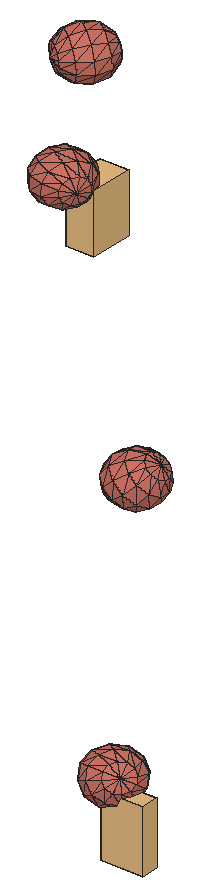
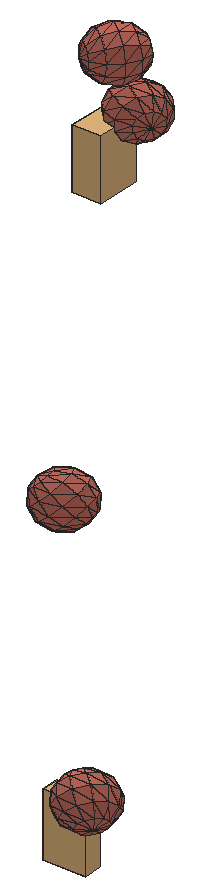
# SketchUp Ruby script. Lengths in inches.
U = 1.inch
M = Sketchup.active_model
def pt(a) = Geom::Point3d.new(a.map { |v| v * U })
def face(e, loops, mat)
  f = e.add_face(loops[0].map { |a| pt(a) })
  loops[1..].each { |l| e.add_face(l.map { |a| pt(a) }).erase! }
  f.material = f.back_material = mat if mat
  f
end
# faces: each face lists its corners as indices into pts; further lists are holes
def faces(e, pts, list, mat = nil) = list.each { |f| face(e, (f[0].is_a?(Array) ? f : [f]).map { |l| l.map { |i| pts[i] } }, mat) }
# xy, xz, yz: faces in a plane at the given z, y or x. An outline is a flat list of corners, or four numbers for a rectangle; further outlines are holes
def ring(l) = l.size == 4 ? [[l[0], l[1]], [l[2], l[1]], [l[2], l[3]], [l[0], l[3]]] : l.each_slice(2).to_a
def flat(e, list, mat, &to3) = list.each { |f| face(e, (f[0].is_a?(Array) ? f : [f]).map { |l| ring(l).map { |u, v| to3.(u, v) } }, mat) }
def xy(e, z, list, mat = nil) = flat(e, list, mat) { |x, y| [x, y, z] }
def xz(e, y, list, mat = nil) = flat(e, list, mat) { |x, z| [x, y, z] }
def yz(e, x, list, mat = nil) = flat(e, list, mat) { |y, z| [x, y, z] }
def lines(e, pts, list) = list.each { |a, b| e.add_line(pt(pts[a]), pt(pts[b])) }
# prism: a flat outline (further loops are holes) pulled along v
def prism(e, loops, v, mat = nil)
  f = face(e, loops, mat); d = Geom::Vector3d.new(v.map { |x| x * U })
  f.pushpull(f.normal.samedirection?(d) ? d.length : -d.length)
end
def box(e, o, s, mat = nil) = prism(e, [[o, [o[0] + s[0], o[1], o[2]], [o[0] + s[0], o[1] + s[1], o[2]], [o[0], o[1] + s[1], o[2]]]], [0, 0, s[2]], mat)
def at(x, y, z, deg = 0) = Geom::Transformation.translation(pt([x, y, z])) * Geom::Transformation.rotation(ORIGIN, Z_AXIS, deg.degrees)
def axes(o, x, y, z) = Geom::Transformation.new([*x, 0, *y, 0, *z, 0, *pt(o).to_a, 1])
def part(name) = M.definitions.add(name)
# library, detail: a bought-in or finely detailed component or shape, given as its bounding box
def library(name, o, s) = part(name).tap { |d| box(d.entities, o, s) }
def detail(e, o, s) = box(e.add_group.entities, o, s)
def put(e, d, t, mat = nil) = e.add_instance(d, t).tap { |i| i.material = mat if mat }
def group(e, t, mat = nil) = e.add_group.tap { |g| g.transformation = t; g.material = mat if mat }.entities
root = M.entities
M.materials.add("green").color = [174, 139, 102]
M.materials.add("vio").color = [206, 114, 100]
c1 = part("3DGeom~208_Defintion")
p = [[-278.9,104.85,-403.93],[-34.22,85.5625,-494.84],[-36.78,-106.97,-488.84],[218.15,-67.8125,-449.7],[219.62,43.35,-453.16],[33.05,253.77,-407.11],
  [-201.22,299.08,-302.625],[-278.9,104.85,-403.93],[-201.22,299.08,-302.625],[-281.85,-117.47,-397],[26.0625,-272.25,-390.72],[254.43,-163.24,-393.05],
  [-278.9,104.85,-403.93],[-281.85,-117.47,-397],[414.62,-10.48,-290.0625],[258.46,140.46,-402.51],[147.02,352.57,-249.16],[-69.62,413.17,-120.23],
  [33.05,253.77,-407.11],[-201.22,299.08,-302.625],[147.02,352.57,-249.16],[33.05,253.77,-407.11],[-448.85,96.04,-204.78],[-278.9,104.85,-403.93],
  [-281.85,-117.47,-397],[-381.57,264.25,-117.05],[-201.22,299.08,-302.625],[258.46,140.46,-402.51],[324.26,197.5,-311.32],[414.62,-10.48,-290.0625],
  [147.02,352.57,-249.16],[324.26,197.5,-311.32],[-451.4,-96.49,-198.78],[-209.29,-308.32,-283.69],[-281.85,-117.47,-397],[-209.29,-308.32,-283.69],
  [318.75,-217.36,-298.39],[318.75,-217.36,-298.39],[254.43,-163.24,-393.05],[414.62,-10.48,-290.0625],[-209.29,-308.32,-283.69],[26.0625,-272.25,-390.72],
  [137.48,-365.99,-226.76],[318.75,-217.36,-298.39],[137.48,-365.99,-226.76],[324.26,197.5,-311.32],[399.39,199.2,-204.01],[414.62,-10.48,-290.0625],
  [277.14,355.5,-63.3],[324.26,197.5,-311.32],[399.39,199.2,-204.01],[324.26,197.5,-311.32],[-267.6,363.06,40.9],[-201.22,299.08,-302.625],
  [-381.57,264.25,-117.05],[-267.6,363.06,40.9],[-201.22,299.08,-302.625],[318.75,-217.36,-298.39],[393.88,-215.66,-191.08],[393.88,-215.66,-191.08],
  [318.75,-217.36,-298.39],[414.62,-10.48,-290.0625],[459.68,-158.62,-99.89],[414.62,-10.48,-290.0625],[498.52,-61.5,-49.24],[414.62,-10.48,-290.0625],
  [500,49.66,-52.7],[414.62,-10.48,-290.0625],[399.39,199.2,-204.01],[463.72,145.08,-109.35],[414.62,-10.48,-290.0625],[414.62,-10.48,-290.0625],
  [-388.56,-261.77,-100.65],[-209.29,-308.32,-283.69],[-80.64,-416.55,-94.37],[-209.29,-308.32,-283.69],[-388.56,-261.77,-100.65],[80.64,416.55,94.37],
  [267.6,-363.06,-40.9],[393.88,-215.66,-191.08],[-498.52,61.5,49.24],[-459.68,158.62,99.89],[388.56,261.77,100.65],[399.39,199.2,-204.01],
  [388.56,261.77,100.65],[399.39,199.2,-204.01],[277.14,355.5,-63.3],[-500,-49.66,52.7],[267.6,-363.06,-40.9],[-137.48,365.99,226.76],
  [-267.6,363.06,40.9],[-393.88,215.66,191.08],[-267.6,363.06,40.9],[451.4,96.49,198.78],[388.56,261.77,100.65],[-388.56,-261.77,-100.65],
  [-277.14,-355.5,63.3],[-463.72,-145.08,109.35],[-277.14,-355.5,63.3],[267.6,-363.06,-40.9],[381.57,-264.25,117.05],[69.62,-413.17,120.23],
  [209.29,308.32,283.69],[388.56,261.77,100.65],[448.85,-96.04,204.78],[381.57,-264.25,117.05],[-318.75,217.36,298.39],[-267.6,363.06,40.9],
  [-393.88,215.66,191.08],[-318.75,217.36,298.39],[-267.6,363.06,40.9],[-414.62,10.48,290.0625],[-147.02,-352.57,249.16],[-277.14,-355.5,63.3],
  [-399.39,-199.2,204.01],[-399.39,-199.2,204.01],[-147.02,-352.57,249.16],[-26.0625,272.25,390.72],[-26.0625,272.25,390.72],[281.85,117.47,397],
  [388.56,261.77,100.65],[281.85,117.47,397],[388.56,261.77,100.65],[209.29,308.32,283.69],[381.57,-264.25,117.05],[201.22,-299.08,302.625],
  [201.22,-299.08,302.625],[-147.02,-352.57,249.16],[201.22,-299.08,302.625],[-318.75,217.36,298.39],[278.9,-104.85,403.93],[278.9,-104.85,403.93],
  [281.85,117.47,397],[-399.39,-199.2,204.01],[-147.02,-352.57,249.16],[-324.26,-197.5,311.32],[-324.26,-197.5,311.32],[201.22,-299.08,302.625],
  [278.9,-104.85,403.93],[-254.43,163.24,393.05],[-137.48,365.99,226.76],[-318.75,217.36,298.39],[-254.43,163.24,393.05],[-26.0625,272.25,390.72],
  [-137.48,365.99,226.76],[-324.26,-197.5,311.32],[-147.02,-352.57,249.16],[-33.05,-253.77,407.11],[-147.02,-352.57,249.16],[201.22,-299.08,302.625],
  [-33.05,-253.77,407.11],[36.78,106.98,488.84],[209.29,308.32,283.69],[281.85,117.47,397],[209.29,308.32,283.69],[-258.46,-140.46,402.51],
  [-258.46,-140.46,402.51],[-219.62,-43.35,453.16],[-414.62,10.48,290.0625],[-218.15,67.8125,449.7],[-414.62,10.48,290.0625],[-254.43,163.24,393.05],
  [-254.43,163.24,393.05],[-414.62,10.48,290.0625],[201.22,-299.08,302.625],[278.9,-104.85,403.93],[-324.26,-197.5,311.32],[-254.43,163.24,393.05],
  [34.22,-85.5625,494.84]]
faces(c1.entities,p,[[0,1,2],[1,3,2],[1,4,3],[5,4,1],[6,1,7],[8,5,1],[9,2,10],[2,11,10],
  [2,3,11],[12,2,13],[3,4,14],[4,15,14],[5,15,4],[11,3,14],[16,15,5],[17,18,19],
  [17,20,21],[22,23,24],[25,23,22],[25,26,23],[27,28,29],[30,31,15],[32,24,33],[34,10,35],
  [22,24,32],[10,11,36],[37,38,39],[40,41,42],[10,43,44],[45,46,47],[48,49,20],[48,50,51],
  [52,53,54],[55,17,56],[42,57,58],[59,60,61],[62,59,63],[64,62,65],[66,64,67],[68,69,70],
  [69,66,71],[72,73,74],[75,42,74],[32,33,76],[77,20,17],[77,48,20],[74,42,78],[42,79,78],
  [80,22,32],[81,22,80],[81,25,22],[82,69,83],[84,85,86],[87,32,76],[80,32,87],[88,59,62],
  [89,17,90],[89,77,17],[91,25,81],[91,92,25],[93,66,69],[93,69,94],[95,74,96],[97,76,98],
  [87,76,97],[99,62,100],[100,62,64],[96,74,101],[74,78,101],[102,103,48],[102,48,77],[104,64,66],
  [104,66,93],[100,64,104],[101,78,105],[106,107,108],[109,89,110],[80,87,111],[81,80,111],[87,97,111],
  [96,101,112],[97,113,114],[115,96,116],[117,77,89],[118,102,77],[91,81,111],[119,93,120],[121,122,123],
  [97,114,111],[101,124,125],[126,100,104],[127,101,128],[129,91,111],[130,104,93],[131,93,132],[133,134,135],
  [114,136,111],[137,104,138],[139,140,141],[142,143,144],[145,146,147],[148,149,150],[151,152,143],[151,153,154],
  [136,155,111],[156,157,158],[157,159,160],[161,129,111],[159,162,163],[147,164,165],[166,147,156],[159,143,167],
  [159,151,143],[168,165,153],[168,153,151],[156,147,168],[156,168,157],[147,165,168],[157,151,159],[157,168,151]],"vio")
c2 = part("3DGeom~244_Defintion")
p = [[-108.99,-83.02,-483.7],[90.05,60.9,-492.09],[201.25,-102.35,-447.625],[393.37,0,-317.28],[-208.69,-14.03,-459.98],[-82.63,180.41,-451.01],
  [264.97,188.51,-368.625],[-44.79,-177.28,-458.03],[-278.83,-204.71,-345.7],[-317.18,11.23,-393.23],[-33.3,-271.53,-389.85],[221.17,-265.61,-329.54],
  [221.17,-265.61,-329.54],[-270.53,224.16,-335.4],[65.57,326.51,-321.2],[416.36,-188.51,-180.93],[221.17,-265.61,-329.54],[416.36,-188.51,-180.93],
  [-405.375,-14.03,-301.34],[-405.375,-14.03,-301.34],[-270.53,224.16,-335.4],[-317.18,11.23,-393.23],[-33.3,-271.53,-389.85],[144.46,-385.12,-169.46],
  [-77.58,-340.53,-297.43],[-33.3,-271.53,-389.85],[221.17,-265.61,-329.54],[-77.58,-340.53,-297.43],[264.97,188.51,-368.625],[480.09,102.35,-101.93],
  [393.37,0,-317.28],[264.97,188.51,-368.625],[368.89,265.61,-146.39],[65.57,326.51,-321.2],[368.89,265.61,-146.39],[264.97,188.51,-368.625],
  [-165.78,-365.79,-205.53],[-165.78,-365.79,-205.53],[-274.26,-340.53,-138.79],[-278.83,-204.71,-345.7],[-274.26,-340.53,-138.79],[-373.96,-271.53,-115.07],
  [-278.83,-204.71,-345.7],[-438.16,-177.28,-140.74],[-278.83,-204.71,-345.7],[-449.66,-83.02,-208.92],[-405.375,-14.03,-301.34],[-278.83,-204.71,-345.7],
  [-278.83,-204.71,-345.7],[-405.375,-14.03,-301.34],[-423.3,180.41,-176.24],[-270.53,224.16,-335.4],[-151.39,377.02,-187.7],[-270.53,224.16,-335.4],
  [-151.39,377.02,-187.7],[327.8,-326.51,3.91],[416.36,-188.51,-180.93],[65.57,326.51,-321.2],[196.2,385.12,-105.3125],[368.89,265.61,-146.39],
  [-151.39,377.02,-187.7],[65.57,326.51,-321.2],[393.37,0,-317.28],[500,-60.9,16.16],[416.36,-188.51,-180.93],[393.37,0,-317.28],
  [-405.375,-14.03,-301.34],[-77.58,-340.53,-297.43],[-8.31,-428.86,-10.3],[-165.78,-365.79,-205.53],[-77.58,-340.53,-297.43],[-500,60.9,-16.16],
  [-165.78,-365.79,-205.53],[-196.2,-385.12,105.3125],[-165.78,-365.79,-205.53],[-274.26,-340.53,-138.79],[-327.8,326.51,-3.91],[-151.39,377.02,-187.7],
  [-327.8,326.51,-3.91],[8.31,428.86,10.3],[-151.39,377.02,-187.7],[-151.39,377.02,-187.7],[416.36,-188.51,-180.93],[423.3,-180.41,176.24],
  [327.8,-326.51,3.91],[416.36,-188.51,-180.93],[151.39,-377.02,187.7],[438.16,177.28,140.74],[373.96,271.53,115.07],[373.96,271.53,115.07],
  [368.89,265.61,-146.39],[-480.09,-102.35,101.93],[-274.26,-340.53,-138.79],[-368.89,-265.61,146.39],[-274.26,-340.53,-138.79],[-368.89,-265.61,146.39],
  [-373.96,-271.53,-115.07],[-368.89,-265.61,146.39],[274.26,340.53,138.79],[373.96,271.53,115.07],[449.66,83.02,208.92],[-416.36,188.51,180.93],
  [-65.57,-326.51,321.2],[-416.36,188.51,180.93],[-144.46,385.12,169.46],[-327.8,326.51,-3.91],[-327.8,326.51,-3.91],[327.8,-326.51,3.91],
  [270.53,-224.16,335.4],[151.39,-377.02,187.7],[327.8,-326.51,3.91],[165.78,365.79,205.53],[405.375,14.03,301.34],[-393.37,0,317.28],
  [-264.97,-188.51,368.625],[-368.89,-265.61,146.39],[-264.97,-188.51,368.625],[278.83,204.71,345.7],[274.26,340.53,138.79],[278.83,204.71,345.7],
  [278.83,204.71,345.7],[278.83,204.71,345.7],[-264.97,-188.51,368.625],[-416.36,188.51,180.93],[-221.17,265.61,329.54],[77.58,340.54,297.43],
  [317.18,-11.23,393.23],[-393.37,0,317.28],[-221.17,265.61,329.54],[-416.36,188.51,180.93],[151.39,-377.02,187.7],[82.63,-180.41,451.01],
  [-65.57,-326.51,321.2],[151.39,-377.02,187.7],[270.53,-224.16,335.4],[165.78,365.79,205.53],[77.58,340.54,297.43],[278.83,204.71,345.7],
  [278.83,204.71,345.7],[77.58,340.54,297.43],[33.3,271.53,389.85],[33.3,271.53,389.85],[317.18,-11.23,393.23],[405.375,14.03,301.34],
  [-264.97,-188.51,368.625],[-201.25,102.35,447.625],[-393.37,0,317.28],[-393.37,0,317.28],[-221.17,265.61,329.54],[-65.57,-326.51,321.2],
  [-90.05,-60.9,492.09],[-264.97,-188.51,368.625],[-65.57,-326.51,321.2],[33.3,271.53,389.85],[-221.17,265.61,329.54],[270.53,-224.16,335.4],
  [208.69,14.03,459.98],[270.53,-224.16,335.4],[317.18,-11.23,393.23],[317.18,-11.23,393.23],[108.99,83.02,483.7],[44.79,177.28,458.03],
  [33.3,271.53,389.85],[-264.97,-188.51,368.625],[33.3,271.53,389.85]]
faces(c2.entities,p,[[0,1,2],[1,3,2],[4,1,0],[4,5,1],[1,6,3],[5,6,1],[0,7,8],[4,0,8],
  [0,2,7],[9,4,8],[9,5,4],[7,10,8],[7,11,10],[7,2,12],[9,13,5],[13,14,5],
  [5,14,6],[2,15,16],[2,3,17],[18,9,8],[19,20,21],[22,23,24],[25,26,23],[10,27,8],
  [28,29,30],[31,32,29],[33,34,35],[27,36,8],[37,38,39],[40,41,42],[41,43,44],[45,46,47],
  [43,45,48],[49,50,51],[50,52,53],[13,54,14],[26,55,23],[26,56,55],[57,58,59],[60,58,61],
  [62,63,64],[65,29,63],[45,50,66],[67,68,69],[70,23,68],[43,71,45],[45,71,50],[72,68,73],
  [74,73,75],[50,76,77],[78,79,80],[81,79,58],[82,83,84],[85,63,83],[71,76,50],[23,86,68],
  [23,55,86],[32,87,29],[32,88,87],[58,89,90],[41,91,43],[43,91,71],[92,73,93],[94,95,96],
  [41,97,91],[58,98,99],[79,98,58],[29,100,63],[29,87,100],[91,101,71],[71,101,76],[68,102,73],
  [68,86,102],[103,104,105],[106,104,79],[107,108,109],[110,83,108],[79,111,98],[104,111,79],[63,112,83],
  [63,100,112],[97,113,91],[91,113,101],[73,114,115],[73,102,116],[87,88,117],[88,118,119],[98,111,120],
  [100,87,121],[97,122,113],[123,124,104],[124,125,104],[104,125,111],[83,126,108],[83,112,126],[127,128,129],
  [130,131,132],[133,134,131],[135,136,137],[112,100,138],[139,140,137],[124,141,125],[142,143,137],[144,145,146],
  [147,145,148],[149,150,151],[152,131,150],[145,153,154],[155,156,131],[157,158,156],[156,159,137],[160,156,137],
  [161,160,137],[162,161,137],[163,150,145],[145,161,164],[150,161,145],[131,160,150],[131,156,160],[150,160,161]],"vio")
c3 = part("3DGeom~248_Defintion")
p = [[242.2,-95.53,-426.77],[-5.12,-61.18,-498.23],[-8.42,49.39,-500],[242.2,-95.53,-426.77],[236.48,95.97,-429.83],[-251.07,-10.43,-436.2],
  [-67.73,144.3,-469.01],[149.39,-262.83,-367.79],[-58.71,-157.77,-464.19],[242.2,-95.53,-426.77],[-167.15,198.125,-413.57],[133.76,260.36,-376.15],
  [133.76,260.36,-376.15],[-17.09,-361.11,-268.71],[-154.82,-214.51,-406.98],[-17.09,-361.11,-268.71],[-267.71,-216.1875,-341.94],[-367.14,-162.36,-286.51],
  [-267.71,-216.1875,-341.94],[-367.14,-162.36,-286.51],[-426.44,-67.45,-255.52],[-426.44,-67.45,-255.52],[-429.75,43.11,-257.28],[-251.07,-10.43,-436.2],
  [-429.75,43.11,-257.28],[-376.16,139.71,-291.33],[-376.16,139.71,-291.33],[-280.04,196.44,-348.54],[-280.04,196.44,-348.54],[424.625,-104.29,-240.95],
  [242.2,-95.53,-426.77],[236.48,95.97,-429.83],[236.48,95.97,-429.83],[418.02,116.84,-244.48],[418.02,116.84,-244.48],[133.76,260.36,-376.15],
  [317.45,-297.47,-172.85],[242.2,-95.53,-426.77],[317.45,-297.47,-172.85],[242.2,-95.53,-426.77],[424.625,-104.29,-240.95],[-38.44,353.59,-280.13],
  [-280.04,196.44,-348.54],[133.76,260.36,-376.15],[-38.44,353.59,-280.13],[-212.625,-364.02,-156.07],[-267.71,-216.1875,-341.94],[-154.82,-214.51,-406.98],
  [-154.82,-214.51,-406.98],[-17.09,-361.11,-268.71],[418.02,116.84,-244.48],[133.76,260.36,-376.15],[299.4,306.66,-182.51],[299.4,306.66,-182.51],
  [133.76,260.36,-376.15],[-38.44,353.59,-280.13],[125.22,-410.95,-58.44],[149.39,-262.83,-367.79],[149.39,-262.83,-367.79],[317.45,-297.47,-172.85],
  [-233.98,350.68,-167.49],[-280.04,196.44,-348.54],[-376.16,139.71,-291.33],[-38.44,353.59,-280.13],[-280.04,196.44,-348.54],[-233.98,350.68,-167.49],
  [-384.83,-270.79,-60.04],[-267.71,-216.1875,-341.94],[-212.625,-364.02,-156.07],[-367.14,-162.36,-286.51],[-267.71,-216.1875,-341.94],[-400.46,252.4,-68.4],
  [-233.98,350.68,-167.49],[-487.55,-106.4,-6.37],[100.5625,414.3125,-71.63],[-233.98,350.68,-167.49],[-100.5625,-414.3125,71.63],[-493.27,85.1,-9.43],
  [493.27,-85.1,9.43],[487.55,106.4,6.37],[299.4,306.66,-182.51],[400.46,-252.4,68.4],[317.45,-297.47,-172.85],[299.4,306.66,-182.51],
  [384.83,270.79,60.04],[384.83,270.79,60.04],[233.98,-350.68,167.49],[317.45,-297.47,-172.85],[233.98,-350.68,167.49],[317.45,-297.47,-172.85],
  [400.46,-252.4,68.4],[-125.22,410.95,58.44],[-400.46,252.4,-68.4],[-299.4,-306.66,182.51],[-299.4,-306.66,182.51],[-384.83,-270.79,-60.04],
  [384.83,270.79,60.04],[212.625,364.02,156.07],[-317.45,297.47,172.85],[-400.46,252.4,-68.4],[-317.45,297.47,172.85],[-418.02,-116.84,244.48],
  [-299.4,-306.66,182.51],[-418.02,-116.84,244.48],[38.44,-353.59,280.13],[38.44,-353.59,280.13],[233.98,-350.68,167.49],[-424.625,104.29,240.95],
  [-317.45,297.47,172.85],[-418.02,-116.84,244.48],[429.75,-43.11,257.28],[426.44,67.45,255.52],[426.44,67.45,255.52],[376.16,-139.71,291.33],
  [376.16,-139.71,291.33],[17.09,361.11,268.71],[-317.45,297.47,172.85],[17.09,361.11,268.71],[426.44,67.45,255.52],[367.14,162.36,286.51],
  [367.14,162.36,286.51],[212.625,364.02,156.07],[280.04,-196.44,348.54],[233.98,-350.68,167.49],[280.04,-196.44,348.54],[376.16,-139.71,291.33],
  [-133.76,-260.36,376.15],[-299.4,-306.66,182.51],[-133.76,-260.36,376.15],[38.44,-353.59,280.13],[367.14,162.36,286.51],[212.625,364.02,156.07],
  [267.71,216.1875,341.94],[267.71,216.1875,341.94],[17.09,361.11,268.71],[167.15,-198.125,413.57],[38.44,-353.59,280.13],[233.98,-350.68,167.49],
  [233.98,-350.68,167.49],[280.04,-196.44,348.54],[-149.39,262.83,367.79],[-317.45,297.47,172.85],[-424.625,104.29,240.95],[17.09,361.11,268.71],
  [-317.45,297.47,172.85],[-149.39,262.83,367.79],[-236.48,-95.97,429.83],[-418.02,-116.84,244.48],[-299.4,-306.66,182.51],[-133.76,-260.36,376.15],
  [-242.2,95.53,426.77],[-418.02,-116.84,244.48],[-424.625,104.29,240.95],[-242.2,95.53,426.77],[-242.2,95.53,426.77],[-418.02,-116.84,244.48],
  [-236.48,-95.97,429.83],[426.44,67.45,255.52],[251.07,10.43,436.2],[426.44,67.45,255.52],[367.14,162.36,286.51],[251.07,10.43,436.2],
  [376.16,-139.71,291.33],[429.75,-43.11,257.28],[154.82,214.51,406.98],[17.09,361.11,268.71],[267.71,216.1875,341.94],[17.09,361.11,268.71],
  [154.82,214.51,406.98],[67.73,-144.3,469.01],[267.71,216.1875,341.94],[58.71,157.77,464.19],[8.42,-49.39,500],[5.12,61.18,498.23]]
faces(c3.entities,p,[[0,1,2],[3,2,4],[2,1,5],[6,2,5],[4,2,6],[7,8,1],[7,1,9],[1,8,5],
  [10,6,5],[4,6,11],[12,6,10],[13,14,8],[15,8,7],[8,14,5],[16,17,5],[14,18,5],
  [19,20,5],[21,22,23],[24,25,5],[26,27,5],[28,10,5],[29,30,31],[29,32,33],[34,4,35],
  [36,7,37],[38,39,40],[41,10,42],[43,10,44],[45,46,47],[45,48,49],[50,51,52],[53,54,55],
  [56,49,57],[56,58,59],[60,61,62],[63,64,65],[66,67,68],[66,69,70],[71,62,22],[72,62,71],
  [73,69,66],[73,21,69],[53,55,74],[74,55,75],[76,45,49],[76,49,56],[77,22,21],[71,22,77],
  [77,21,73],[78,29,33],[78,33,79],[79,33,80],[81,82,29],[81,29,78],[79,83,84],[85,53,74],
  [86,56,87],[88,89,90],[91,75,92],[74,75,91],[93,45,76],[94,95,45],[96,74,97],[97,74,91],
  [98,71,77],[91,99,100],[101,66,102],[103,73,66],[104,76,56],[105,56,106],[107,77,73],[108,77,107],
  [107,73,109],[110,78,79],[110,79,111],[112,79,84],[113,81,78],[114,78,110],[115,91,116],[97,91,117],
  [118,84,119],[120,84,121],[122,123,81],[124,81,125],[126,127,76],[128,76,129],[130,131,132],[133,97,134],
  [135,136,137],[135,138,139],[140,141,142],[143,144,145],[146,147,148],[146,148,149],[150,107,151],[140,152,153],
  [154,155,156],[110,157,158],[159,160,161],[162,163,161],[164,165,140],[166,167,168],[169,149,136],[169,136,135],
  [160,170,161],[139,162,161],[170,164,161],[135,139,161],[171,140,153],[164,140,171],[172,146,149],[172,149,169],
  [164,171,161],[169,135,161],[173,153,146],[171,153,173],[173,146,172],[172,169,161],[173,172,161],[171,173,161]],"vio")
c4 = part("3DGeom~241_Defintion")
p = [[-83.63,87.77,-500],[-95.35,-182.17,-461.02],[-273.19,-13.21,-439.1],[14.09,-123.87,-496.18],[142.8125,124.74,-475.08],[-158.95,275.9,-369.85],
  [-273.19,-13.21,-439.1],[102.53,318.58,-341.07],[-158.95,275.9,-369.85],[102.53,318.58,-341.07],[108.04,-302.32,-359.41],[144.83,-102.53,-481.79],
  [108.04,-302.32,-359.41],[261.83,-123.87,-421.71],[108.04,-302.32,-359.41],[345.47,87.77,-371.01],[336.53,275.9,-220.9],[336.53,275.9,-220.9],
  [102.53,318.58,-341.07],[-154.17,-261.82,-385.73],[108.04,-302.32,-359.41],[-273.19,-13.21,-439.1],[-273.19,-13.21,-439.1],[-375.08,-151.16,-308.7],
  [-377.83,159.29,-299.52],[-273.19,-13.21,-439.1],[-375.08,-151.16,-308.7],[-158.95,275.9,-369.85],[-273.19,-13.21,-439.1],[-377.83,159.29,-299.52],
  [333.75,-182.17,-332.03],[108.04,-302.32,-359.41],[470.03,-13.21,-215.68],[333.75,-182.17,-332.03],[261.83,-123.87,-421.71],[261.83,-123.87,-421.71],
  [345.47,87.77,-371.01],[-375.08,-151.16,-308.7],[-146.61,-341.47,-290.49],[-146.61,-341.47,-290.49],[108.04,-302.32,-359.41],[480.36,159.29,-41.54],
  [345.47,87.77,-371.01],[345.47,87.77,-371.01],[336.53,275.9,-220.9],[-191.67,390.1,-140.59],[-158.95,275.9,-369.85],[34.77,427.0625,-115.67],
  [-158.95,275.9,-369.85],[-191.67,390.1,-140.59],[102.53,318.58,-341.07],[-158.95,275.9,-369.85],[42.3,-421.11,-140.72],[-74.7,-399.77,-200.81],
  [108.04,-302.32,-359.41],[173.04,-399.77,-126.33],[-146.61,-341.47,-290.49],[282.49,-341.47,-161.49],[341.31,-261.82,-236.78],[282.49,-341.47,-161.49],
  [333.75,-182.17,-332.03],[341.31,-261.82,-236.78],[108.04,-302.32,-359.41],[237.42,390.1,-11.6],[336.53,275.9,-220.9],[483.12,-151.16,-50.71],
  [341.31,-261.82,-236.78],[-375.08,-151.16,-308.7],[-146.61,-341.47,-290.49],[-361.98,-289.11,-143.73],[-495.48,0,-148.95],[-361.98,-289.11,-143.73],
  [-381.24,289.11,-79.69],[-191.67,390.1,-140.59],[-361.98,-289.11,-143.73],[381.24,-289.11,79.69],[282.49,-341.47,-161.49],[361.98,289.11,143.73],
  [336.53,275.9,-220.9],[361.98,289.11,143.73],[336.53,275.9,-220.9],[237.42,390.1,-11.6],[495.48,0,148.95],[-237.42,-390.1,11.6],
  [-361.98,-289.11,-143.73],[191.67,-390.1,140.59],[282.49,-341.47,-161.49],[191.67,-390.1,140.59],[282.49,-341.47,-161.49],[381.24,-289.11,79.69],
  [-480.36,-159.29,41.54],[-483.12,151.16,50.71],[-237.42,-390.1,11.6],[-34.77,-427.0625,115.67],[-173.04,399.77,126.33],[-381.24,289.11,-79.69],
  [-42.3,421.11,140.72],[191.67,-390.1,140.59],[74.7,399.77,200.81],[-282.49,341.47,161.5],[-381.24,289.11,-79.69],[-282.49,341.47,161.5],
  [377.83,-159.29,299.53],[375.08,151.16,308.7],[375.08,151.16,308.7],[361.98,289.11,143.73],[146.61,341.47,290.49],[361.98,289.11,143.73],
  [-336.53,-275.9,220.9],[-237.42,-390.1,11.6],[-336.53,-275.9,220.9],[-470.03,13.21,215.68],[-336.53,-275.9,220.9],[-341.31,261.82,236.78],
  [-282.49,341.47,161.5],[-341.31,261.82,236.78],[158.95,-275.9,369.85],[191.67,-390.1,140.59],[158.95,-275.9,369.85],[-336.53,-275.9,220.9],
  [-102.53,-318.58,341.07],[-102.53,-318.58,341.07],[191.67,-390.1,140.59],[-108.04,302.32,359.41],[-108.04,302.32,359.41],[-102.53,-318.58,341.07],
  [191.67,-390.1,140.59],[158.95,-275.9,369.85],[-108.04,302.32,359.41],[154.17,261.82,385.73],[375.08,151.16,308.7],[361.98,289.11,143.73],
  [361.98,289.11,143.73],[146.61,341.47,290.49],[273.19,13.21,439.1],[273.19,13.21,439.1],[375.08,151.16,308.7],[-341.31,261.82,236.78],
  [-108.04,302.32,359.41],[-108.04,302.32,359.41],[-336.53,-275.9,220.9],[-345.47,-87.77,371.01],[-333.75,182.17,332.03],[-345.47,-87.77,371.01],
  [-341.31,261.82,236.78],[-333.75,182.17,332.03],[-345.47,-87.77,371.01],[-336.53,-275.9,220.9],[-102.53,-318.58,341.07],[-341.31,261.82,236.78],
  [-333.75,182.17,332.03],[-108.04,302.32,359.41],[146.61,341.47,290.49],[83.63,-87.77,500],[158.95,-275.9,369.85],[377.83,-159.29,299.53],
  [377.83,-159.29,299.53],[273.19,13.21,439.1],[95.35,182.17,461.02],[-333.75,182.17,332.03],[-345.47,-87.77,371.01],[-261.83,123.87,421.71],
  [-261.83,123.87,421.71],[-142.8125,-124.74,475.08],[-144.83,102.53,481.79],[-14.09,123.87,496.18]]
faces(c4.entities,p,[[0,1,2],[0,3,1],[4,3,0],[5,0,6],[7,0,8],[9,4,0],[1,3,10],[3,11,12],
  [4,11,3],[11,13,14],[15,13,11],[15,11,4],[16,15,4],[17,4,18],[19,1,20],[21,1,19],
  [22,19,23],[24,25,26],[27,28,29],[13,30,31],[32,33,34],[32,35,36],[37,19,38],[39,19,40],
  [41,32,42],[41,43,44],[45,46,24],[47,48,49],[47,50,51],[52,53,54],[55,52,54],[53,56,54],
  [57,55,54],[58,59,54],[60,61,62],[63,64,50],[63,50,47],[65,66,33],[65,33,32],[67,68,69],
  [70,26,71],[24,26,70],[72,24,70],[73,24,72],[74,56,53],[75,76,66],[75,66,65],[77,41,78],
  [79,80,81],[82,65,32],[82,32,41],[83,53,52],[84,53,83],[85,55,86],[87,88,89],[70,71,90],
  [91,70,90],[72,70,91],[90,71,92],[83,52,93],[93,52,55],[94,49,95],[96,47,49],[96,49,94],
  [93,55,97],[98,63,47],[98,47,96],[99,72,91],[94,100,101],[102,75,65],[102,65,82],[103,82,41],
  [104,41,105],[106,107,63],[106,63,98],[108,83,93],[90,109,110],[111,90,112],[91,90,111],[113,91,111],
  [114,91,115],[116,117,75],[118,75,102],[119,93,120],[121,93,122],[94,101,123],[96,94,124],[125,126,127],
  [98,96,128],[129,130,131],[129,132,133],[134,102,82],[135,82,136],[101,137,138],[106,98,139],[111,140,141],
  [142,111,143],[144,111,145],[146,147,148],[149,150,151],[129,152,151],[153,154,155],[153,156,157],[158,157,130],
  [158,130,129],[159,160,161],[150,162,151],[146,148,163],[163,148,154],[162,164,151],[164,165,151],[165,158,151],
  [158,129,151],[163,154,153],[162,146,163],[162,163,164],[165,153,157],[165,157,158],[164,163,153],[164,153,165]],"vio")
c5 = library("3DGeom~173_Defintion",[-146.02,-500,-341.01],[292.04,1000,682.02])
c6 = part("3DGeom~174_Defintion")
p = [[-127.07,494.74,-302.98],[-83.38,461.51,-336.48],[-100.9,461.46,-341.01],[-127.07,494.74,-302.98],[-117.78,466.57,-338.44],[-127.07,494.74,-302.98],
  [-117.78,466.57,-338.44],[-129.48,475.47,-329.47],[-127.07,494.74,-302.98],[-69.91,466.72,-326.0625],[-127.07,494.74,-302.98],[-129.48,475.47,-329.47],
  [-132.89,485.78,-316.49],[-127.07,494.74,-302.98],[-64.09,475.68,-312.56],[-69.91,466.72,-326.0625],[-127.07,494.74,-302.98],[-67.49,485.99,-299.58],
  [-64.09,475.68,-312.56],[-127.07,494.74,-302.98],[-79.2,494.89,-290.61],[-67.49,485.99,-299.58],[-127.07,494.74,-302.98],[-113.59,499.94,-292.57],
  [-96.07,500,-288.04],[-127.07,494.74,-302.98],[-96.07,500,-288.04],[-79.2,494.89,-290.61],[109.52,-498.77,278.33],[81.81,-497.43,299.58],
  [93.08,-500,285.75],[109.52,-498.77,278.33],[84.66,-484.5,330.92],[81.81,-497.43,299.58],[140.09,-487.18,288.41],[84.66,-484.5,330.92],
  [109.52,-498.77,278.33],[140.09,-487.18,288.41],[109.52,-498.77,278.33],[126.73,-494.08,279.3],[142.9375,-474.24,319.75],[84.66,-484.5,330.92],
  [140.09,-487.18,288.41],[142.9375,-474.24,319.75],[140.09,-487.18,288.41],[146.02,-479.92,303.22],[84.66,-484.5,330.92],[78.73,-491.76,316.12],
  [81.81,-497.43,299.58],[115.22,-472.9,341.01],[84.66,-484.5,330.92],[142.9375,-474.24,319.75],[115.22,-472.9,341.01],[142.9375,-474.24,319.75],
  [131.66,-471.68,333.58],[84.66,-484.5,330.92],[115.22,-472.9,341.01],[98.02,-477.6,340.03]]
faces(c6.entities,p,[[0,1,2],[3,2,4],[5,6,7],[8,9,1],[10,11,12],[13,14,15],[16,17,18],[19,20,21],
  [22,23,24],[25,26,27],[28,29,30],[31,32,33],[34,35,36],[37,38,39],[40,41,42],[43,44,45],
  [46,47,48],[49,50,51],[52,53,54],[55,56,57]],"green")
c7 = library("3DGeom~181_Defintion",[-363.49,-500,-241.625],[726.98,1000,483.25])
c8 = part("3DGeom~182_Defintion")
p = [[358.51,487.39,-222.91],[326.92,489.88,-241.625],[308.78,492.93,-236.98],[358.51,487.39,-222.91],[345.12,487.85,-236.47],[326.92,489.88,-241.625],
  [358.51,487.39,-222.91],[308.78,492.93,-236.98],[295.57,496.1875,-223.79],[358.51,487.39,-222.91],[295.57,496.1875,-223.79],[290.82,498.77,-205.58],
  [358.51,487.39,-222.91],[290.82,498.77,-205.58],[295.8,500,-187.23],[358.51,487.39,-222.91],[295.8,500,-187.23],[309.18,499.54,-173.67],
  [358.51,487.39,-222.91],[309.18,499.54,-173.67],[327.38,497.51,-168.51],[358.51,487.39,-222.91],[327.38,497.51,-168.51],[345.52,494.46,-173.16],
  [358.51,487.39,-222.91],[345.52,494.46,-173.16],[358.74,491.2,-186.35],[358.51,487.39,-222.91],[358.74,491.2,-186.35],[363.49,488.61,-204.5625],
  [-336.99,-490.37,173.04],[-308.93,-500,194.02],[-361.3125,-469.79,186.35],[-308.93,-500,194.02],[-336.99,-490.37,173.04],[-321.37,-497.625,179.85],
  [-336.99,-490.37,173.04],[-361.3125,-469.79,186.35],[-351.61,-480.18,175.42],[-361.3125,-469.79,186.35],[-308.93,-500,194.02],[-357.5625,-458.84,220.65],
  [-361.3125,-469.79,186.35],[-357.5625,-458.84,220.65],[-363.49,-461.98,202.91],[-357.5625,-458.84,220.65],[-308.93,-500,194.02],[-329.5,-468.47,241.625],
  [-329.5,-468.47,241.625],[-308.93,-500,194.02],[-305.18,-489.05,228.31],[-308.93,-500,194.02],[-303,-496.86,211.76],[-305.18,-489.05,228.31],
  [-357.5625,-458.84,220.65],[-329.5,-468.47,241.625],[-345.12,-461.21,234.82],[-329.5,-468.47,241.625],[-305.18,-489.05,228.31],[-314.88,-478.66,239.24]]
faces(c8.entities,p,[[0,1,2],[3,4,5],[6,7,8],[9,10,11],[12,13,14],[15,16,17],[18,19,20],[21,22,23],
  [24,25,26],[27,28,29],[30,31,32],[33,34,35],[36,37,38],[39,40,41],[42,43,44],[45,46,47],
  [48,49,50],[51,52,53],[54,55,56],[57,58,59]],"green")
g1 = group(root,at(15.3125,38.42,26.21))
put(g1,c1,axes([-1.55,-0.47,14.8],[0,0.00039,0],[0,0,-0.00039],[-0.00039,0,0]),"vio")
g2 = group(root,at(15.3125,38.42,26.21))
put(g2,c2,axes([-1.47,-0.33,10.38],[0,0.00039,0],[0,0,-0.00039],[-0.00039,0,0]),"vio")
g3 = group(root,at(15.3125,38.42,26.21))
put(g3,c3,axes([-1.41,-0.83,14.25],[0,0.00039,0],[0,0,-0.00039],[-0.00039,0,0]),"vio")
g4 = group(root,at(15.3125,38.42,26.21))
put(g4,c4,axes([-1.38,-0.25,12.18],[0,0.00038,0],[0,0,-0.00038],[-0.00038,0,0]),"vio")
g5 = group(root,at(15.3125,38.42,26.21))
put(g5,c5,axes([-1.32,-0.39,10.14],[0,0.00042,0],[0,0,-0.00042],[-0.00042,0,0]),"green")
put(g5,c6,axes([-1.32,-0.39,10.14],[0,0.00042,0],[0,0,-0.00042],[-0.00042,0,0]),"green")
g6 = group(root,at(15.3125,38.42,26.21))
put(g6,c7,axes([-1.31,-0.67,14.03],[0,0.0004,0],[0,0,-0.0004],[-0.0004,0,0]),"green")
put(g6,c8,axes([-1.31,-0.67,14.03],[0,0.0004,0],[0,0,-0.0004],[-0.0004,0,0]),"green")
